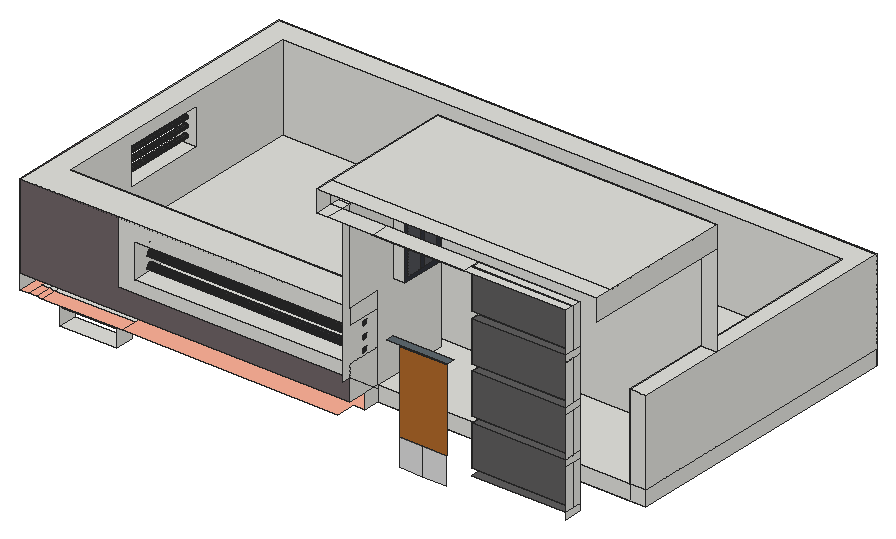
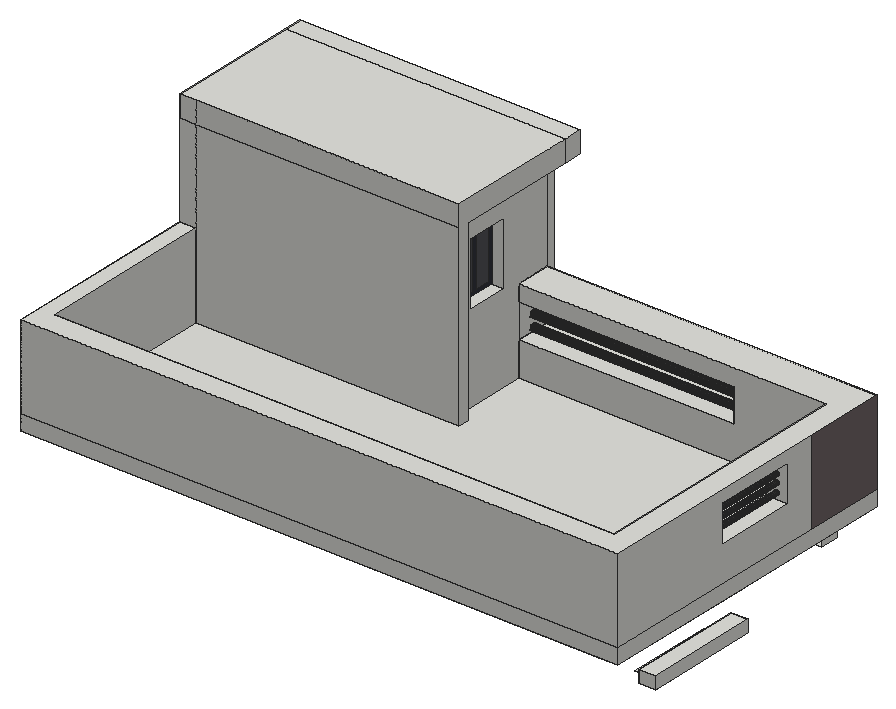
# SketchUp Ruby script. Lengths in inches.
U = 1.inch
M = Sketchup.active_model
def pt(a) = Geom::Point3d.new(a.map { |v| v * U })
def face(e, loops, mat)
  f = e.add_face(loops[0].map { |a| pt(a) })
  loops[1..].each { |l| e.add_face(l.map { |a| pt(a) }).erase! }
  f.material = f.back_material = mat if mat
  f
end
# faces: each face lists its corners as indices into pts; further lists are holes
def faces(e, pts, list, mat = nil) = list.each { |f| face(e, (f[0].is_a?(Array) ? f : [f]).map { |l| l.map { |i| pts[i] } }, mat) }
# xy, xz, yz: faces in a plane at the given z, y or x. An outline is a flat list of corners, or four numbers for a rectangle; further outlines are holes
def ring(l) = l.size == 4 ? [[l[0], l[1]], [l[2], l[1]], [l[2], l[3]], [l[0], l[3]]] : l.each_slice(2).to_a
def flat(e, list, mat, &to3) = list.each { |f| face(e, (f[0].is_a?(Array) ? f : [f]).map { |l| ring(l).map { |u, v| to3.(u, v) } }, mat) }
def xy(e, z, list, mat = nil) = flat(e, list, mat) { |x, y| [x, y, z] }
def xz(e, y, list, mat = nil) = flat(e, list, mat) { |x, z| [x, y, z] }
def yz(e, x, list, mat = nil) = flat(e, list, mat) { |y, z| [x, y, z] }
def lines(e, pts, list) = list.each { |a, b| e.add_line(pt(pts[a]), pt(pts[b])) }
# prism: a flat outline (further loops are holes) pulled along v
def prism(e, loops, v, mat = nil)
  f = face(e, loops, mat); d = Geom::Vector3d.new(v.map { |x| x * U })
  f.pushpull(f.normal.samedirection?(d) ? d.length : -d.length)
end
def box(e, o, s, mat = nil) = prism(e, [[o, [o[0] + s[0], o[1], o[2]], [o[0] + s[0], o[1] + s[1], o[2]], [o[0], o[1] + s[1], o[2]]]], [0, 0, s[2]], mat)
def at(x, y, z, deg = 0) = Geom::Transformation.translation(pt([x, y, z])) * Geom::Transformation.rotation(ORIGIN, Z_AXIS, deg.degrees)
def axes(o, x, y, z) = Geom::Transformation.new([*x, 0, *y, 0, *z, 0, *pt(o).to_a, 1])
def part(name) = M.definitions.add(name)
# library, detail: a bought-in or finely detailed component or shape, given as its bounding box
def library(name, o, s) = part(name).tap { |d| box(d.entities, o, s) }
def detail(e, o, s) = box(e.add_group.entities, o, s)
def put(e, d, t, mat = nil) = e.add_instance(d, t).tap { |i| i.material = mat if mat }
def group(e, t, mat = nil) = e.add_group.tap { |g| g.transformation = t; g.material = mat if mat }.entities
root = M.entities
M.materials.add("[Asphalt New]").color = [112, 100, 103]
M.materials.add("[Blinds Roman Hobbled Blue]").color = [81, 82, 87]
M.materials.add("[Color B02]").color = [255, 178, 153]
M.materials.add("[Color M07]").color = [58, 58, 58]
M.materials.add("[Formica Laminate Dark]").color = [50, 53, 60]
M.materials.add("[Formica Speckled Grey]").color = [94, 105, 111]
M.materials.add("[Granite Dark Gray]").color = [96, 95, 95]
M.materials.add("[Translucent Glass Gray]").color = [128, 128, 128]
M.materials["[Translucent Glass Gray]"].alpha = 0.5
M.materials.add("[Wood Bamboo]").color = [177, 105, 43]
box(root,[0,145.22,293.87],[9.125,62.75,6.5])
xy(root,292.4,[[23.59,55.96,54.34,66.17]])
xy(root,293.4,[[9.125,153.59,17.5,199.9]])
xy(root,301.78,[[23.59,55.96,54.34,66.17]])
xy(root,308.75,[[13.5,55.96,17.87,66.17],[17.87,55.96,20.93,66.17],[20.93,55.96,64.52,66.17],[323.83,66.17,332.57,132.14],[9.125,132.14,323.83,139.76],
  [323.83,132.14,332.57,139.76],[9.125,139.76,17.87,222.09],[17.87,139.76,323.83,213.34],[323.83,139.76,332.57,222.09],[17.87,213.34,323.83,222.09]])
xy(root,308.75,[[9.125,47.05,9.125,132.14,323.83,132.14,323.83,66.17,187.4,66.17,187.4,57.43,181.15,57.43,181.15,47.05,64.52,47.05,64.52,66.17,13.5,66.17,13.5,47.05],[13.5,47.05,17.87,55.96],[17.87,47.05,20.93,55.96],[20.93,47.05,64.52,55.96]],"[Color B02]")
xy(root,311.4375,[[261.16,37.37,315.98,42.24]],"[Granite Dark Gray]")
xy(root,314.99,[[261.16,37.37,315.98,42.24]],"[Granite Dark Gray]")
xy(root,316.8125,[[9.125,47.05,9.125,222.09,332.57,222.09,332.57,66.17,323.83,66.17,323.83,209.67,21.01,209.67,21.01,66.17,187.4,66.17,187.4,47.05],[21.01,66.17,187.4,66.17,187.4,108.53,181.33,108.53,181.33,114.05,323.83,114.05,323.83,209.67,21.01,209.67],[187.4,66.17,323.83,66.17,323.83,114.05,181.33,114.05,181.33,108.53,187.4,108.53]])
xy(root,335.45,[[70.91,47.05,187.4,66.17]])
xy(root,336.27,[[9.125,106.83,21.01,151.83]])
xy(root,336.8125,[[261.16,37.37,315.98,42.24]],"[Granite Dark Gray]")
xy(root,340.37,[[261.16,37.37,315.98,42.24]],"[Granite Dark Gray]")
xy(root,353.69,[[70.91,47.05,187.4,66.17]])
xy(root,356.33,[[9.125,106.83,21.01,151.83]])
xy(root,362.1875,[[261.16,37.37,315.98,42.24]],"[Granite Dark Gray]")
xy(root,362.75,[[9.125,47.05,187.4,47.05,187.4,66.17,21.01,66.17,21.01,209.67,323.83,209.67,323.83,114.05,332.57,114.05,332.57,222.09,9.125,222.09],[323.83,66.17,332.57,114.05]])
xy(root,364.47,[[187.4,76.04,194.02,99.54]])
xy(root,364.92,[[219.35,32.05,252.53,36.24]],"[Formica Speckled Grey]")
xy(root,365.74,[[261.16,37.37,315.98,42.24]],"[Granite Dark Gray]")
xy(root,387.5625,[[261.16,37.37,315.98,42.24]],"[Granite Dark Gray]")
xy(root,391.12,[[261.16,37.37,315.98,42.24]],"[Granite Dark Gray]")
xy(root,398.97,[[187.4,76.04,194.02,99.54]])
xy(root,412.9375,[[211.57,32.05,261.16,32.62],[181.33,32.62,187.4,42.24],[187.4,32.62,211.57,42.24],[211.57,32.62,261.16,42.24],[261.16,32.62,315.98,37.37],
  [261.16,37.37,315.98,42.24],[181.33,42.24,187.4,47.05],[181.33,47.05,187.4,108.53]])
xy(root,424.6875,[[181.33,32.62,332.57,42.24],[181.33,42.24,332.57,114.05]])
xz(root,36.24,[[223.21,302.2,235.94,317.34],[235.94,302.2,248.67,317.34]],"[Translucent Glass Gray]")
xz(root,36.24,[[223.21,317.34,248.67,361.06]],"[Wood Bamboo]")
xz(root,37.37,[[261.16,314.99,315.98,336.8125],[261.16,340.37,315.98,362.1875],[261.16,365.74,315.98,387.5625],[261.16,391.12,315.98,412.9375]],"[Granite Dark Gray]")
xz(root,42.24,[[261.16,314.99,315.98,336.8125],[261.16,340.37,315.98,362.1875],[261.16,365.74,315.98,387.5625],[261.16,391.12,315.98,412.9375]])
xz(root,42.24,[[261.16,311.4375,315.98,314.99],[261.16,336.8125,315.98,340.37],[261.16,362.1875,315.98,365.74],[261.16,387.5625,315.98,391.12]],"[Formica Laminate Dark]")
xz(root,47.05,[[62.58,328.8125,187.4,328.8125,187.4,335.45,70.91,335.45,70.91,353.69,187.4,353.69,187.4,362.75,62.58,362.75]])
xz(root,47.05,[[9.125,316.8125,187.4,316.8125,187.4,328.8125,62.58,328.8125,62.58,362.75,9.125,362.75]],"[Asphalt New]")
xz(root,66.17,[[187.4,308.75,323.83,316.8125],[323.83,308.75,332.57,316.8125],[21.01,316.8125,21.01,362.75,187.4,362.75,187.4,353.69,70.91,353.69,70.91,335.45,187.4,335.45,187.4,316.8125],[323.83,316.8125,332.57,362.75]])
xz(root,76.04,[[187.4,364.47,194.02,398.97]])
xz(root,99.54,[[187.4,364.47,194.02,398.97]])
xz(root,106.83,[[[9.125,336.27,21.01,356.33],[15.03,352.34,15.34,352.38,15.63,352.5,15.875,352.68,16.0625,352.93,16.18,353.22,16.22,353.52,16.18,353.83,16.0625,354.12,15.875,354.36,15.63,354.55,15.34,354.67,15.03,354.71,14.73,354.67,14.44,354.55,14.19,354.36,14.01,354.12,13.89,353.83,13.85,353.52,13.89,353.22,14.01,352.93,14.19,352.68,14.44,352.5,14.73,352.38],[15.03,347.84,15.34,347.88,15.63,348,15.875,348.18,16.0625,348.43,16.18,348.72,16.22,349.02,16.18,349.33,16.0625,349.62,15.875,349.86,15.63,350.05,15.34,350.17,15.03,350.21,14.73,350.17,14.44,350.05,14.19,349.86,14.01,349.62,13.89,349.33,13.85,349.02,13.89,348.72,14.01,348.43,14.19,348.18,14.44,348,14.73,347.88],[15.03,338.46,15.34,338.5,15.63,338.62,15.875,338.81,16.0625,339.06,16.18,339.34,16.22,339.65,16.18,339.96,16.0625,340.24,15.875,340.49,15.63,340.68,15.34,340.8,15.03,340.84,14.73,340.8,14.44,340.68,14.19,340.49,14.01,340.24,13.89,339.96,13.85,339.65,13.89,339.34,14.01,339.06,14.19,338.81,14.44,338.62,14.73,338.5],[15.03,343.34,15.34,343.38,15.63,343.5,15.875,343.68,16.0625,343.93,16.18,344.22,16.22,344.52,16.18,344.83,16.0625,345.12,15.875,345.36,15.63,345.55,15.34,345.67,15.03,345.71,14.73,345.67,14.44,345.55,14.19,345.36,14.01,345.12,13.89,344.83,13.85,344.52,13.89,344.22,14.01,343.93,14.19,343.68,14.44,343.5,14.73,343.38]]])
xz(root,108.53,[[181.33,316.8125,187.4,412.9375]])
xz(root,114.05,[[181.33,316.8125,323.83,412.9375],[323.83,362.75,332.57,412.9375],[181.33,412.9375,323.83,424.6875],[323.83,412.9375,332.57,424.6875]])
xz(root,151.83,[[[9.125,336.27,21.01,356.33],[15.03,338.46,14.73,338.5,14.44,338.62,14.19,338.81,14.01,339.06,13.89,339.34,13.85,339.65,13.89,339.96,14.01,340.24,14.19,340.49,14.44,340.68,14.73,340.8,15.03,340.84,15.34,340.8,15.63,340.68,15.875,340.49,16.0625,340.24,16.18,339.96,16.22,339.65,16.18,339.34,16.0625,339.06,15.875,338.81,15.63,338.62,15.34,338.5],[15.03,352.34,14.73,352.38,14.44,352.5,14.19,352.68,14.01,352.93,13.89,353.22,13.85,353.52,13.89,353.83,14.01,354.12,14.19,354.36,14.44,354.55,14.73,354.67,15.03,354.71,15.34,354.67,15.63,354.55,15.875,354.36,16.0625,354.12,16.18,353.83,16.22,353.52,16.18,353.22,16.0625,352.93,15.875,352.68,15.63,352.5,15.34,352.38],[15.03,347.84,14.73,347.88,14.44,348,14.19,348.18,14.01,348.43,13.89,348.72,13.85,349.02,13.89,349.33,14.01,349.62,14.19,349.86,14.44,350.05,14.73,350.17,15.03,350.21,15.34,350.17,15.63,350.05,15.875,349.86,16.0625,349.62,16.18,349.33,16.22,349.02,16.18,348.72,16.0625,348.43,15.875,348.18,15.63,348,15.34,347.88],[15.03,343.34,14.73,343.38,14.44,343.5,14.19,343.68,14.01,343.93,13.89,344.22,13.85,344.52,13.89,344.83,14.01,345.12,14.19,345.36,14.44,345.55,14.73,345.67,15.03,345.71,15.34,345.67,15.63,345.55,15.875,345.36,16.0625,345.12,16.18,344.83,16.22,344.52,16.18,344.22,16.0625,343.93,15.875,343.68,15.63,343.5,15.34,343.38]],[15.03,338.46,14.73,338.5,14.44,338.62,14.19,338.81,14.01,339.06,13.89,339.34,13.85,339.65,13.89,339.96,14.01,340.24,14.19,340.49,14.44,340.68,14.73,340.8,15.03,340.84,15.34,340.8,15.63,340.68,15.875,340.49,16.0625,340.24,16.18,339.96,16.22,339.65,16.18,339.34,16.0625,339.06,15.875,338.81,15.63,338.62,15.34,338.5],[15.03,343.34,14.73,343.38,14.44,343.5,14.19,343.68,14.01,343.93,13.89,344.22,13.85,344.52,13.89,344.83,14.01,345.12,14.19,345.36,14.44,345.55,14.73,345.67,15.03,345.71,15.34,345.67,15.63,345.55,15.875,345.36,16.0625,345.12,16.18,344.83,16.22,344.52,16.18,344.22,16.0625,343.93,15.875,343.68,15.63,343.5,15.34,343.38],[15.03,347.84,14.73,347.88,14.44,348,14.19,348.18,14.01,348.43,13.89,348.72,13.85,349.02,13.89,349.33,14.01,349.62,14.19,349.86,14.44,350.05,14.73,350.17,15.03,350.21,15.34,350.17,15.63,350.05,15.875,349.86,16.0625,349.62,16.18,349.33,16.22,349.02,16.18,348.72,16.0625,348.43,15.875,348.18,15.63,348,15.34,347.88],[15.03,352.34,14.73,352.38,14.44,352.5,14.19,352.68,14.01,352.93,13.89,353.22,13.85,353.52,13.89,353.83,14.01,354.12,14.19,354.36,14.44,354.55,14.73,354.67,15.03,354.71,15.34,354.67,15.63,354.55,15.875,354.36,16.0625,354.12,16.18,353.83,16.22,353.52,16.18,353.22,16.0625,352.93,15.875,352.68,15.63,352.5,15.34,352.38]])
xz(root,209.67,[[21.01,316.8125,323.83,362.75]])
xz(root,222.09,[[9.125,308.75,332.57,316.8125],[9.125,316.8125,332.57,362.75]])
yz(root,9.125,[[47.05,308.75,222.09,316.8125],[[91.71,316.8125,222.09,362.75],[106.83,336.27,151.83,356.33]]])
yz(root,9.125,[[47.05,316.8125,91.71,362.75]],"[Asphalt New]")
yz(root,21.01,[[[66.17,316.8125,209.67,362.75],[106.83,336.27,151.83,356.33]]])
yz(root,23.59,[[55.96,292.4,66.17,301.78]])
yz(root,54.34,[[55.96,292.4,66.17,301.78]])
yz(root,70.91,[[[47.05,335.45,66.17,353.69],[57.16,336.15,56.7,336.21,56.28,336.39,55.92,336.66,55.64,337.03,55.47,337.45,55.41,337.9,55.47,338.36,55.64,338.78,55.92,339.14,56.28,339.42,56.7,339.59,57.16,339.65,57.61,339.59,58.03,339.42,58.39,339.14,58.67,338.78,58.85,338.36,58.91,337.9,58.85,337.45,58.67,337.03,58.39,336.66,58.03,336.39,57.61,336.21],[57.16,349.28,56.7,349.34,56.28,349.51,55.92,349.79,55.64,350.15,55.47,350.57,55.41,351.03,55.47,351.48,55.64,351.9,55.92,352.26,56.28,352.54,56.7,352.72,57.16,352.78,57.61,352.72,58.03,352.54,58.39,352.26,58.67,351.9,58.85,351.48,58.91,351.03,58.85,350.57,58.67,350.15,58.39,349.79,58.03,349.51,57.61,349.34],[57.16,342.53,56.7,342.59,56.28,342.76,55.92,343.04,55.64,343.4,55.47,343.82,55.41,344.28,55.47,344.73,55.64,345.15,55.92,345.51,56.28,345.79,56.7,345.97,57.16,346.03,57.61,345.97,58.03,345.79,58.39,345.51,58.67,345.15,58.85,344.73,58.91,344.28,58.85,343.82,58.67,343.4,58.39,343.04,58.03,342.76,57.61,342.59]],[57.16,336.15,56.7,336.21,56.28,336.39,55.92,336.66,55.64,337.03,55.47,337.45,55.41,337.9,55.47,338.36,55.64,338.78,55.92,339.14,56.28,339.42,56.7,339.59,57.16,339.65,57.61,339.59,58.03,339.42,58.39,339.14,58.67,338.78,58.85,338.36,58.91,337.9,58.85,337.45,58.67,337.03,58.39,336.66,58.03,336.39,57.61,336.21],[57.16,342.53,56.7,342.59,56.28,342.76,55.92,343.04,55.64,343.4,55.47,343.82,55.41,344.28,55.47,344.73,55.64,345.15,55.92,345.51,56.28,345.79,56.7,345.97,57.16,346.03,57.61,345.97,58.03,345.79,58.39,345.51,58.67,345.15,58.85,344.73,58.91,344.28,58.85,343.82,58.67,343.4,58.39,343.04,58.03,342.76,57.61,342.59],[57.16,349.28,56.7,349.34,56.28,349.51,55.92,349.79,55.64,350.15,55.47,350.57,55.41,351.03,55.47,351.48,55.64,351.9,55.92,352.26,56.28,352.54,56.7,352.72,57.16,352.78,57.61,352.72,58.03,352.54,58.39,352.26,58.67,351.9,58.85,351.48,58.91,351.03,58.85,350.57,58.67,350.15,58.39,349.79,58.03,349.51,57.61,349.34]])
yz(root,181.33,[[108.53,316.8125,108.53,412.9375,42.24,412.9375,42.24,424.6875,114.05,424.6875,114.05,316.8125],[32.62,412.9375,42.24,424.6875]])
yz(root,187.4,[[57.43,308.75,66.17,316.8125],[47.05,316.8125,66.17,335.45],[[66.17,316.8125,66.17,362.75,47.05,362.75,47.05,412.9375,108.53,412.9375,108.53,316.8125],[76.04,364.47,99.54,398.97]],[[42.24,328.8125,42.24,412.9375,47.05,412.9375,47.05,353.69,66.17,353.69,66.17,335.45,47.05,335.45,47.05,328.8125],[57.16,349.28,57.61,349.34,58.03,349.51,58.39,349.79,58.67,350.15,58.85,350.57,58.91,351.03,58.85,351.48,58.67,351.9,58.39,352.26,58.03,352.54,57.61,352.72,57.16,352.78,56.7,352.72,56.28,352.54,55.92,352.26,55.64,351.9,55.47,351.48,55.41,351.03,55.47,350.57,55.64,350.15,55.92,349.79,56.28,349.51,56.7,349.34],[57.16,342.53,57.61,342.59,58.03,342.76,58.39,343.04,58.67,343.4,58.85,343.82,58.91,344.28,58.85,344.73,58.67,345.15,58.39,345.51,58.03,345.79,57.61,345.97,57.16,346.03,56.7,345.97,56.28,345.79,55.92,345.51,55.64,345.15,55.47,344.73,55.41,344.28,55.47,343.82,55.64,343.4,55.92,343.04,56.28,342.76,56.7,342.59],[57.16,336.15,57.61,336.21,58.03,336.39,58.39,336.66,58.67,337.03,58.85,337.45,58.91,337.9,58.85,338.36,58.67,338.78,58.39,339.14,58.03,339.42,57.61,339.59,57.16,339.65,56.7,339.59,56.28,339.42,55.92,339.14,55.64,338.78,55.47,338.36,55.41,337.9,55.47,337.45,55.64,337.03,55.92,336.66,56.28,336.39,56.7,336.21]],[47.05,353.69,66.17,362.75]])
yz(root,194.02,[[78.02,366.45,87.28,396.99],[88.89,366.45,97.55,396.99]],"[Blinds Roman Hobbled Blue]")
yz(root,194.02,[[[76.04,364.47,99.54,398.97],[78.02,366.45,97.55,396.99]],[87.28,366.45,88.89,396.99]],"[Formica Laminate Dark]")
yz(root,261.16,[[37.37,314.99,42.24,336.8125],[37.37,340.37,42.24,362.1875],[37.37,365.74,42.24,387.5625],[37.37,391.12,42.24,412.9375]])
yz(root,315.98,[[32.62,311.4375,42.24,314.99],[32.62,314.99,37.37,336.8125],[37.37,314.99,42.24,336.8125],[32.62,336.8125,42.24,340.37],[32.62,340.37,37.37,362.1875],
  [37.37,340.37,42.24,362.1875],[32.62,362.1875,42.24,365.74],[32.62,365.74,37.37,387.5625],[37.37,365.74,42.24,387.5625],[32.62,387.5625,42.24,391.12],
  [32.62,391.12,37.37,412.9375],[37.37,391.12,42.24,412.9375]])
yz(root,323.83,[[66.17,316.8125,114.05,362.75],[114.05,316.8125,209.67,362.75]])
yz(root,332.57,[[66.17,308.75,222.09,316.8125],[66.17,316.8125,222.09,362.75],[32.62,412.9375,114.05,424.6875]])
p = [[70.91,56.28,336.39],[70.91,56.7,336.21],[187.4,56.7,336.21],[187.4,56.28,336.39],[70.91,57.16,336.15],[187.4,57.16,336.15],
  [70.91,57.61,336.21],[187.4,57.61,336.21],[70.91,58.03,336.39],[187.4,58.03,336.39],[70.91,55.92,336.66],[187.4,55.92,336.66],
  [70.91,58.39,336.66],[187.4,58.39,336.66],[70.91,55.64,337.03],[187.4,55.64,337.03],[70.91,58.67,337.03],[187.4,58.67,337.03],
  [70.91,55.47,337.45],[187.4,55.47,337.45],[70.91,58.85,337.45],[187.4,58.85,337.45],[70.91,55.41,337.9],[187.4,55.41,337.9],
  [70.91,58.91,337.9],[187.4,58.91,337.9],[70.91,55.47,338.36],[187.4,55.47,338.36],[70.91,58.85,338.36],[187.4,58.85,338.36],
  [70.91,55.64,338.78],[187.4,55.64,338.78],[70.91,58.67,338.78],[187.4,58.67,338.78],[14.44,151.83,338.62],[14.73,151.83,338.5],
  [14.73,106.83,338.5],[14.44,106.83,338.62],[15.03,151.83,338.46],[15.03,106.83,338.46],[15.34,151.83,338.5],[15.34,106.83,338.5],
  [15.63,151.83,338.62],[15.63,106.83,338.62],[14.19,151.83,338.81],[14.19,106.83,338.81],[15.875,151.83,338.81],[15.875,106.83,338.81],
  [70.91,55.92,339.14],[187.4,55.92,339.14],[70.91,58.39,339.14],[187.4,58.39,339.14],[14.01,151.83,339.06],[14.01,106.83,339.06],
  [16.0625,151.83,339.06],[16.0625,106.83,339.06],[70.91,56.28,339.42],[187.4,56.28,339.42],[70.91,58.03,339.42],[187.4,58.03,339.42],
  [13.89,151.83,339.34],[13.89,106.83,339.34],[16.18,151.83,339.34],[16.18,106.83,339.34],[13.85,151.83,339.65],[13.85,106.83,339.65],
  [16.22,151.83,339.65],[16.22,106.83,339.65],[70.91,56.7,339.59],[187.4,56.7,339.59],[70.91,57.61,339.59],[187.4,57.61,339.59],
  [70.91,57.16,339.65],[187.4,57.16,339.65],[13.89,151.83,339.96],[13.89,106.83,339.96],[16.18,151.83,339.96],[16.18,106.83,339.96],
  [14.01,151.83,340.24],[14.01,106.83,340.24],[16.0625,151.83,340.24],[16.0625,106.83,340.24],[14.19,151.83,340.49],[14.19,106.83,340.49],
  [15.875,151.83,340.49],[15.875,106.83,340.49],[14.44,151.83,340.68],[14.44,106.83,340.68],[15.63,151.83,340.68],[15.63,106.83,340.68],
  [14.73,151.83,340.8],[14.73,106.83,340.8],[15.34,151.83,340.8],[15.34,106.83,340.8],[15.03,151.83,340.84],[15.03,106.83,340.84],
  [70.91,56.7,342.59],[70.91,57.16,342.53],[187.4,57.16,342.53],[187.4,56.7,342.59],[70.91,57.61,342.59],[187.4,57.61,342.59],
  [70.91,56.28,342.76],[187.4,56.28,342.76],[70.91,58.03,342.76],[187.4,58.03,342.76],[70.91,55.92,343.04],[187.4,55.92,343.04],
  [70.91,58.39,343.04],[187.4,58.39,343.04],[70.91,55.64,343.4],[187.4,55.64,343.4],[70.91,58.67,343.4],[187.4,58.67,343.4],
  [14.73,151.83,343.38],[15.03,151.83,343.34],[15.03,106.83,343.34],[14.73,106.83,343.38],[15.34,151.83,343.38],[15.34,106.83,343.38],
  [70.91,55.47,343.82],[187.4,55.47,343.82],[70.91,58.85,343.82],[187.4,58.85,343.82],[14.44,151.83,343.5],[14.44,106.83,343.5],
  [15.63,151.83,343.5],[15.63,106.83,343.5],[14.19,151.83,343.68],[14.19,106.83,343.68],[15.875,151.83,343.68],[15.875,106.83,343.68],
  [14.01,151.83,343.93],[14.01,106.83,343.93],[16.0625,151.83,343.93],[16.0625,106.83,343.93],[70.91,55.41,344.28],[187.4,55.41,344.28],
  [70.91,58.91,344.28],[187.4,58.91,344.28],[13.89,151.83,344.22],[13.89,106.83,344.22],[16.18,151.83,344.22],[16.18,106.83,344.22],
  [13.85,151.83,344.52],[13.85,106.83,344.52],[16.22,151.83,344.52],[16.22,106.83,344.52],[70.91,55.47,344.73],[187.4,55.47,344.73],
  [70.91,58.85,344.73],[187.4,58.85,344.73],[13.89,151.83,344.83],[13.89,106.83,344.83],[16.18,151.83,344.83],[16.18,106.83,344.83],
  [70.91,55.64,345.15],[187.4,55.64,345.15],[70.91,58.67,345.15],[187.4,58.67,345.15],[14.01,151.83,345.12],[14.01,106.83,345.12],
  [16.0625,151.83,345.12],[16.0625,106.83,345.12],[14.19,151.83,345.36],[14.19,106.83,345.36],[15.875,151.83,345.36],[15.875,106.83,345.36],
  [70.91,55.92,345.51],[187.4,55.92,345.51],[70.91,58.39,345.51],[187.4,58.39,345.51],[14.44,151.83,345.55],[14.44,106.83,345.55],
  [15.63,151.83,345.55],[15.63,106.83,345.55],[70.91,56.28,345.79],[187.4,56.28,345.79],[70.91,58.03,345.79],[187.4,58.03,345.79],
  [14.73,151.83,345.67],[14.73,106.83,345.67],[15.34,151.83,345.67],[15.34,106.83,345.67],[15.03,151.83,345.71],[15.03,106.83,345.71],
  [70.91,56.7,345.97],[187.4,56.7,345.97],[70.91,57.61,345.97],[187.4,57.61,345.97],[70.91,57.16,346.03],[187.4,57.16,346.03],
  [14.73,151.83,347.88],[15.03,151.83,347.84],[15.03,106.83,347.84],[14.73,106.83,347.88],[15.34,151.83,347.88],[15.34,106.83,347.88],
  [14.44,151.83,348],[14.44,106.83,348],[15.63,151.83,348],[15.63,106.83,348],[14.19,151.83,348.18],[14.19,106.83,348.18],
  [15.875,151.83,348.18],[15.875,106.83,348.18],[14.01,151.83,348.43],[14.01,106.83,348.43],[16.0625,151.83,348.43],[16.0625,106.83,348.43],
  [13.89,151.83,348.72],[13.89,106.83,348.72],[16.18,151.83,348.72],[16.18,106.83,348.72],[13.85,151.83,349.02],[13.85,106.83,349.02],
  [16.22,151.83,349.02],[16.22,106.83,349.02],[13.89,151.83,349.33],[13.89,106.83,349.33],[16.18,151.83,349.33],[16.18,106.83,349.33],
  [70.91,56.28,349.51],[70.91,56.7,349.34],[187.4,56.7,349.34],[187.4,56.28,349.51],[70.91,57.16,349.28],[187.4,57.16,349.28],
  [70.91,57.61,349.34],[187.4,57.61,349.34],[70.91,58.03,349.51],[187.4,58.03,349.51],[14.01,151.83,349.62],[14.01,106.83,349.62],
  [16.0625,151.83,349.62],[16.0625,106.83,349.62],[70.91,55.92,349.79],[187.4,55.92,349.79],[70.91,58.39,349.79],[187.4,58.39,349.79],
  [14.19,151.83,349.86],[14.19,106.83,349.86],[15.875,151.83,349.86],[15.875,106.83,349.86],[70.91,55.64,350.15],[187.4,55.64,350.15],
  [70.91,58.67,350.15],[187.4,58.67,350.15],[14.44,151.83,350.05],[14.44,106.83,350.05],[15.63,151.83,350.05],[15.63,106.83,350.05],
  [14.73,151.83,350.17],[14.73,106.83,350.17],[15.34,151.83,350.17],[15.34,106.83,350.17],[70.91,55.47,350.57],[187.4,55.47,350.57],
  [70.91,58.85,350.57],[187.4,58.85,350.57],[15.03,151.83,350.21],[15.03,106.83,350.21],[70.91,55.41,351.03],[187.4,55.41,351.03],
  [70.91,58.91,351.03],[187.4,58.91,351.03],[70.91,55.47,351.48],[187.4,55.47,351.48],[70.91,58.85,351.48],[187.4,58.85,351.48],
  [70.91,55.64,351.9],[187.4,55.64,351.9],[70.91,58.67,351.9],[187.4,58.67,351.9],[70.91,55.92,352.26],[187.4,55.92,352.26],
  [70.91,58.39,352.26],[187.4,58.39,352.26],[70.91,56.28,352.54],[187.4,56.28,352.54],[70.91,58.03,352.54],[187.4,58.03,352.54],
  [14.73,151.83,352.38],[15.03,151.83,352.34],[15.03,106.83,352.34],[14.73,106.83,352.38],[15.34,151.83,352.38],[15.34,106.83,352.38],
  [14.44,151.83,352.5],[14.44,106.83,352.5],[15.63,151.83,352.5],[15.63,106.83,352.5],[70.91,56.7,352.72],[187.4,56.7,352.72],
  [70.91,57.61,352.72],[187.4,57.61,352.72],[14.19,151.83,352.68],[14.19,106.83,352.68],[15.875,151.83,352.68],[15.875,106.83,352.68],
  [70.91,57.16,352.78],[187.4,57.16,352.78],[14.01,151.83,352.93],[14.01,106.83,352.93],[16.0625,151.83,352.93],[16.0625,106.83,352.93],
  [13.89,151.83,353.22],[13.89,106.83,353.22],[16.18,151.83,353.22],[16.18,106.83,353.22],[13.85,151.83,353.52],[13.85,106.83,353.52],
  [16.22,151.83,353.52],[16.22,106.83,353.52],[13.89,151.83,353.83],[13.89,106.83,353.83],[16.18,151.83,353.83],[16.18,106.83,353.83],
  [14.01,151.83,354.12],[14.01,106.83,354.12],[16.0625,151.83,354.12],[16.0625,106.83,354.12],[14.19,151.83,354.36],[14.19,106.83,354.36],
  [15.875,151.83,354.36],[15.875,106.83,354.36],[14.44,151.83,354.55],[14.44,106.83,354.55],[15.63,151.83,354.55],[15.63,106.83,354.55],
  [14.73,151.83,354.67],[14.73,106.83,354.67],[15.34,151.83,354.67],[15.34,106.83,354.67],[15.03,151.83,354.71],[15.03,106.83,354.71],
  [187.4,47.05,328.8125],[200.02,47.05,328.8125],[202.71,47.05,328.8125]]
faces(root,p,[[0,1,2,3],[1,4,5,2],[4,6,7,5],[6,8,9,7],[10,0,3,11],[8,12,13,9],[14,10,11,15],[12,16,17,13],
  [18,14,15,19],[16,20,21,17],[22,18,19,23],[20,24,25,21],[26,22,23,27],[24,28,29,25],[30,26,27,31],[28,32,33,29],
  [34,35,36,37],[35,38,39,36],[38,40,41,39],[40,42,43,41],[44,34,37,45],[42,46,47,43],[48,30,31,49],[32,50,51,33],
  [52,44,45,53],[46,54,55,47],[56,48,49,57],[50,58,59,51],[60,52,53,61],[54,62,63,55],[64,60,61,65],[62,66,67,63],
  [68,56,57,69],[58,70,71,59],[72,68,69,73],[70,72,73,71],[74,64,65,75],[66,76,77,67],[78,74,75,79],[76,80,81,77],
  [82,78,79,83],[80,84,85,81],[86,82,83,87],[84,88,89,85],[90,86,87,91],[88,92,93,89],[94,90,91,95],[92,94,95,93],
  [96,97,98,99],[97,100,101,98],[102,96,99,103],[100,104,105,101],[106,102,103,107],[104,108,109,105],[110,106,107,111],[108,112,113,109],
  [114,115,116,117],[115,118,119,116],[120,110,111,121],[112,122,123,113],[124,114,117,125],[118,126,127,119],[128,124,125,129],[126,130,131,127],
  [132,128,129,133],[130,134,135,131],[136,120,121,137],[122,138,139,123],[140,132,133,141],[134,142,143,135],[144,140,141,145],[142,146,147,143],
  [148,136,137,149],[138,150,151,139],[152,144,145,153],[146,154,155,147],[156,148,149,157],[150,158,159,151],[160,152,153,161],[154,162,163,155],
  [164,160,161,165],[162,166,167,163],[168,156,157,169],[158,170,171,159],[172,164,165,173],[166,174,175,167],[176,168,169,177],[170,178,179,171],
  [180,172,173,181],[174,182,183,175],[184,180,181,185],[182,184,185,183],[186,176,177,187],[178,188,189,179],[190,186,187,191],[188,190,191,189],
  [192,193,194,195],[193,196,197,194],[198,192,195,199],[196,200,201,197],[202,198,199,203],[200,204,205,201],[206,202,203,207],[204,208,209,205],
  [210,206,207,211],[208,212,213,209],[214,210,211,215],[212,216,217,213],[218,214,215,219],[216,220,221,217],[222,223,224,225],[223,226,227,224],
  [226,228,229,227],[228,230,231,229],[232,218,219,233],[220,234,235,221],[236,222,225,237],[230,238,239,231],[240,232,233,241],[234,242,243,235],
  [244,236,237,245],[238,246,247,239],[248,240,241,249],[242,250,251,243],[252,248,249,253],[250,254,255,251],[256,244,245,257],[246,258,259,247],
  [260,252,253,261],[254,260,261,255],[262,256,257,263],[258,264,265,259],[266,262,263,267],[264,268,269,265],[270,266,267,271],[268,272,273,269],
  [274,270,271,275],[272,276,277,273],[278,274,275,279],[276,280,281,277],[282,283,284,285],[283,286,287,284],[288,282,285,289],[286,290,291,287],
  [292,278,279,293],[280,294,295,281],[296,288,289,297],[290,298,299,291],[300,292,293,301],[294,300,301,295],[302,296,297,303],[298,304,305,299],
  [306,302,303,307],[304,308,309,305],[310,306,307,311],[308,312,313,309],[314,310,311,315],[312,316,317,313],[318,314,315,319],[316,320,321,317],
  [322,318,319,323],[320,324,325,321],[326,322,323,327],[324,328,329,325],[330,326,327,331],[328,332,333,329],[334,330,331,335],[332,334,335,333]],"[Color M07]")
lines(root,p,[[336,337],[337,338]])
